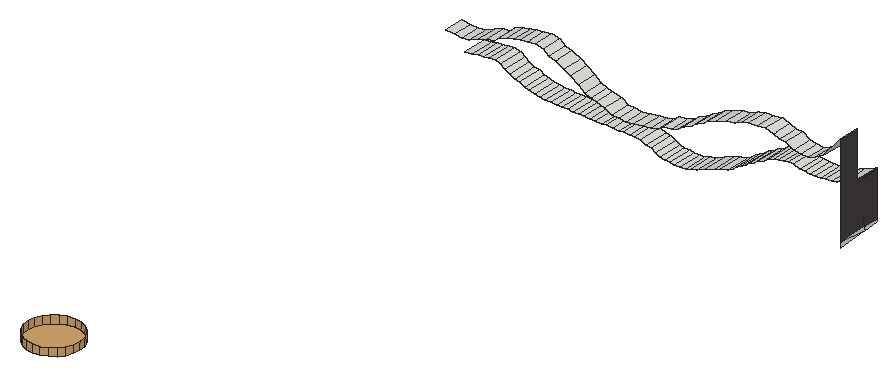
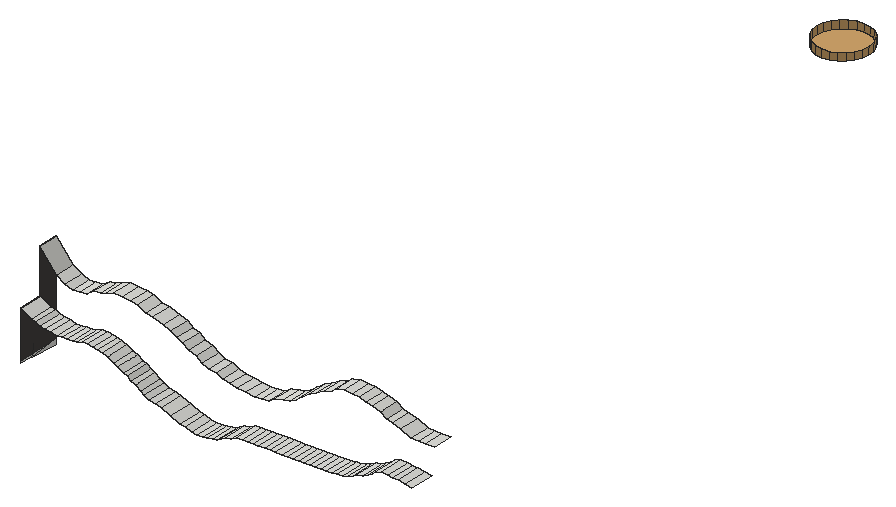
# SketchUp Ruby script. Lengths in inches.
U = 1.inch
M = Sketchup.active_model
def pt(a) = Geom::Point3d.new(a.map { |v| v * U })
def face(e, loops, mat)
  f = e.add_face(loops[0].map { |a| pt(a) })
  loops[1..].each { |l| e.add_face(l.map { |a| pt(a) }).erase! }
  f.material = f.back_material = mat if mat
  f
end
# faces: each face lists its corners as indices into pts; further lists are holes
def faces(e, pts, list, mat = nil) = list.each { |f| face(e, (f[0].is_a?(Array) ? f : [f]).map { |l| l.map { |i| pts[i] } }, mat) }
# xy, xz, yz: faces in a plane at the given z, y or x. An outline is a flat list of corners, or four numbers for a rectangle; further outlines are holes
def ring(l) = l.size == 4 ? [[l[0], l[1]], [l[2], l[1]], [l[2], l[3]], [l[0], l[3]]] : l.each_slice(2).to_a
def flat(e, list, mat, &to3) = list.each { |f| face(e, (f[0].is_a?(Array) ? f : [f]).map { |l| ring(l).map { |u, v| to3.(u, v) } }, mat) }
def xy(e, z, list, mat = nil) = flat(e, list, mat) { |x, y| [x, y, z] }
def xz(e, y, list, mat = nil) = flat(e, list, mat) { |x, z| [x, y, z] }
def yz(e, x, list, mat = nil) = flat(e, list, mat) { |y, z| [x, y, z] }
def lines(e, pts, list) = list.each { |a, b| e.add_line(pt(pts[a]), pt(pts[b])) }
# prism: a flat outline (further loops are holes) pulled along v
def prism(e, loops, v, mat = nil)
  f = face(e, loops, mat); d = Geom::Vector3d.new(v.map { |x| x * U })
  f.pushpull(f.normal.samedirection?(d) ? d.length : -d.length)
end
def box(e, o, s, mat = nil) = prism(e, [[o, [o[0] + s[0], o[1], o[2]], [o[0] + s[0], o[1] + s[1], o[2]], [o[0], o[1] + s[1], o[2]]]], [0, 0, s[2]], mat)
def at(x, y, z, deg = 0) = Geom::Transformation.translation(pt([x, y, z])) * Geom::Transformation.rotation(ORIGIN, Z_AXIS, deg.degrees)
def axes(o, x, y, z) = Geom::Transformation.new([*x, 0, *y, 0, *z, 0, *pt(o).to_a, 1])
def part(name) = M.definitions.add(name)
# library, detail: a bought-in or finely detailed component or shape, given as its bounding box
def library(name, o, s) = part(name).tap { |d| box(d.entities, o, s) }
def detail(e, o, s) = box(e.add_group.entities, o, s)
def put(e, d, t, mat = nil) = e.add_instance(d, t).tap { |i| i.material = mat if mat }
def group(e, t, mat = nil) = e.add_group.tap { |g| g.transformation = t; g.material = mat if mat }.entities
root = M.entities
M.materials.add("[Field Square Tile]").color = [211, 167, 108]
M.materials.add("[Granite Tile]1").color = [68, 65, 63]
xy(root,250.6875,[[2134.543,2328.207,2133.831,2328.3,2133.168,2328.575,2132.598,2329.012,2132.161,2329.582,2131.886,2330.245,2131.793,2330.957,2131.886,2331.668,2132.161,2332.332,2132.598,2332.901,2133.168,2333.338,2133.831,2333.613,2134.543,2333.707,2135.254,2333.613,2135.918,2333.338,2136.487,2332.901,2136.924,2332.332,2137.199,2331.668,2137.293,2330.957,2137.199,2330.245,2136.924,2329.582,2136.487,2329.012,2135.918,2328.575,2135.254,2328.3]],"[Field Square Tile]")
yz(root,2164.345,[[2396.678,240.932,2396.678,241.519,2399.776,241.17],[2399.81,241.167,2399.776,241.17,2399.809,241.173],[2399.776,241.17,2396.678,241.519,2399.769,241.519,2399.809,241.173],[2399.809,241.173,2399.769,241.519,2401.365,241.519,2401.365,241.293]])
yz(root,2164.345,[[2396.678,241.519,2396.678,251.165,2398.803,251.165,2398.803,246.426,2401.365,246.426,2401.365,241.519]],"[Granite Tile]1")
p = [[2144.767,2398.803,241.17],[2144.767,2401.365,241.17],[2145.237,2401.365,241.121],[2145.237,2398.803,241.121],[2145.843,2401.365,241.09],[2145.843,2398.803,241.09],
  [2146.41,2401.365,241.138],[2146.41,2398.803,241.138],[2147.05,2401.365,241.346],[2147.05,2398.803,241.346],[2143.769,2398.803,241.332],[2143.769,2401.365,241.332],
  [2144.237,2401.365,241.243],[2144.237,2398.803,241.243],[2143.35,2398.803,241.566],[2143.35,2401.365,241.566],[2147.641,2401.365,241.456],[2147.641,2398.803,241.456],
  [2148.576,2401.365,241.847],[2148.576,2398.803,241.847],[2142.844,2398.803,241.837],[2142.844,2401.365,241.837],[2142.271,2398.803,241.967],[2142.271,2401.365,241.967],
  [2149.581,2401.365,242.229],[2149.581,2398.803,242.229],[2141.69,2398.803,242.199],[2141.69,2401.365,242.199],[2141.064,2398.803,242.277],[2141.064,2401.365,242.277],
  [2150.142,2401.365,242.424],[2150.142,2398.803,242.424],[2135.217,2398.803,242.35],[2135.217,2401.365,242.35],[2135.799,2401.365,242.342],[2135.799,2398.803,242.342],
  [2136.381,2401.365,242.334],[2136.381,2398.803,242.334],[2136.963,2401.365,242.326],[2136.963,2398.803,242.326],[2137.683,2401.365,242.317],[2137.683,2398.803,242.317],
  [2138.153,2401.365,242.312],[2138.153,2398.803,242.312],[2138.794,2401.365,242.304],[2138.794,2398.803,242.304],[2139.458,2401.365,242.296],[2139.458,2398.803,242.296],
  [2139.91,2401.365,242.291],[2139.91,2398.803,242.291],[2140.548,2401.365,242.283],[2140.548,2398.803,242.283],[2131.735,2398.803,242.466],[2131.735,2401.365,242.466],
  [2132.311,2401.365,242.428],[2132.311,2398.803,242.428],[2132.89,2401.365,242.403],[2132.89,2398.803,242.403],[2133.47,2401.365,242.385],[2133.47,2398.803,242.385],
  [2134.052,2401.365,242.371],[2134.052,2398.803,242.371],[2134.634,2401.365,242.36],[2134.634,2398.803,242.36],[2150.86,2401.365,242.605],[2150.86,2398.803,242.605],
  [2130.607,2398.803,242.599],[2130.607,2401.365,242.599],[2131.167,2401.365,242.518],[2131.167,2398.803,242.518],[2130.054,2398.803,242.75],[2130.054,2401.365,242.75],
  [2151.373,2401.365,242.907],[2151.373,2398.803,242.907],[2129.566,2398.803,242.921],[2129.566,2401.365,242.921],[2129.075,2398.803,243.216],[2129.075,2401.365,243.216],
  [2151.745,2401.365,243.144],[2151.745,2398.803,243.144],[2152.294,2401.365,243.516],[2152.294,2398.803,243.516],[2128.527,2398.803,243.332],[2128.527,2401.365,243.332],
  [2127.982,2398.803,243.589],[2127.982,2401.365,243.589],[2152.768,2401.365,243.711],[2152.768,2398.803,243.711],[2127.501,2398.803,243.88],[2127.501,2401.365,243.88],
  [2153.099,2401.365,244.02],[2153.099,2398.803,244.02],[2127.124,2398.803,244.194],[2127.124,2401.365,244.194],[2123.336,2398.803,243.992],[2123.336,2401.365,243.992],
  [2124.039,2401.365,244.076],[2124.039,2398.803,244.076],[2153.543,2401.365,244.206],[2153.543,2398.803,244.206],[2124.738,2401.365,244.207],[2124.738,2398.803,244.207],
  [2125.323,2401.365,244.266],[2125.323,2398.803,244.266],[2126.527,2398.803,244.387],[2126.527,2401.365,244.387],[2154.132,2401.365,244.569],[2154.132,2398.803,244.569],
  [2125.864,2401.365,244.296],[2125.864,2398.803,244.296],[2154.602,2401.365,244.757],[2154.602,2398.803,244.757],[2155.219,2401.365,245.125],[2155.219,2398.803,245.125],
  [2140.415,2396.678,245.064],[2140.415,2398.803,245.064],[2141.125,2398.803,244.949],[2141.125,2396.678,244.949],[2141.839,2398.803,244.867],[2141.839,2396.678,244.867],
  [2142.745,2398.803,245.007],[2142.745,2396.678,245.007],[2143.689,2398.803,245.121],[2143.689,2396.678,245.121],[2139.702,2396.678,245.459],[2139.702,2398.803,245.459],
  [2144.454,2398.803,245.254],[2144.454,2396.678,245.254],[2155.723,2401.365,245.32],[2155.723,2398.803,245.32],[2159.424,2398.803,245.272],[2159.424,2401.365,245.272],
  [2159.982,2401.365,245.235],[2159.982,2398.803,245.235],[2160.536,2401.365,245.216],[2160.536,2398.803,245.216],[2161.101,2401.365,245.34],[2161.101,2398.803,245.34],
  [2145.206,2398.803,245.41],[2145.206,2396.678,245.41],[2156.205,2401.365,245.411],[2156.205,2398.803,245.411],[2157.771,2398.803,245.552],[2157.771,2401.365,245.552],
  [2158.379,2401.365,245.346],[2158.379,2398.803,245.346],[2158.873,2401.365,245.309],[2158.873,2398.803,245.309],[2161.733,2401.365,245.423],[2161.733,2398.803,245.423],
  [2145.84,2398.803,245.775],[2145.84,2396.678,245.775],[2156.753,2401.365,245.481],[2156.753,2398.803,245.481],[2162.311,2401.365,245.516],[2162.311,2398.803,245.516],
  [2138.827,2396.678,245.671],[2138.827,2398.803,245.671],[2157.235,2401.365,245.59],[2157.235,2398.803,245.59],[2162.691,2401.365,245.763],[2162.691,2398.803,245.763],
  [2138.152,2396.678,245.834],[2138.152,2398.803,245.834],[2137.564,2396.678,246.129],[2137.564,2398.803,246.129],[2146.636,2398.803,245.88],[2146.636,2396.678,245.88],
  [2163.16,2401.365,245.896],[2163.16,2398.803,245.896],[2147.349,2398.803,246.16],[2147.349,2396.678,246.16],[2164.345,2401.365,246.426],[2164.345,2398.803,246.426],
  [2136.933,2396.678,246.633],[2136.933,2398.803,246.633],[2147.946,2398.803,246.573],[2147.946,2396.678,246.573],[2136.119,2396.678,247.185],[2136.119,2398.803,247.185],
  [2148.736,2398.803,246.902],[2148.736,2396.678,246.902],[2123.942,2396.678,246.79],[2123.942,2398.803,246.79],[2124.721,2398.803,246.747],[2124.721,2396.678,246.747],
  [2125.468,2398.803,246.831],[2125.468,2396.678,246.831],[2122.988,2396.678,246.838],[2122.988,2398.803,246.838],[2126.51,2398.803,247.251],[2126.51,2396.678,247.251],
  [2149.338,2398.803,247.347],[2149.338,2396.678,247.347],[2135.407,2396.678,247.553],[2135.407,2398.803,247.553],[2127.384,2398.803,247.546],[2127.384,2396.678,247.546],
  [2150.012,2398.803,247.615],[2150.012,2396.678,247.615],[2128.046,2398.803,247.657],[2128.046,2396.678,247.657],[2134.516,2396.678,248.059],[2134.516,2398.803,248.059],
  [2150.599,2398.803,248.057],[2150.599,2396.678,248.057],[2128.679,2398.803,248.162],[2128.679,2396.678,248.162],[2133.825,2396.678,248.257],[2133.825,2398.803,248.257],
  [2151.364,2398.803,248.322],[2151.364,2396.678,248.322],[2129.473,2398.803,248.408],[2129.473,2396.678,248.408],[2160.161,2396.678,248.295],[2160.161,2398.803,248.295],
  [2160.87,2398.803,248.218],[2160.87,2396.678,248.218],[2161.687,2398.803,248.558],[2161.687,2396.678,248.558],[2133.294,2396.678,248.687],[2133.294,2398.803,248.687],
  [2152.475,2398.803,248.655],[2152.475,2396.678,248.655],[2159.45,2396.678,248.42],[2159.45,2398.803,248.42],[2130.172,2398.803,248.521],[2130.172,2396.678,248.521],
  [2158.653,2396.678,248.895],[2158.653,2398.803,248.895],[2130.866,2398.803,248.723],[2130.866,2396.678,248.723],[2162.622,2398.803,249.022],[2162.622,2396.678,249.022],
  [2131.565,2398.803,248.801],[2131.565,2396.678,248.801],[2132.462,2396.678,248.851],[2132.462,2398.803,248.851],[2153.248,2398.803,248.795],[2153.248,2396.678,248.795],
  [2154.111,2398.803,249.194],[2154.111,2396.678,249.194],[2157.949,2396.678,248.962],[2157.949,2398.803,248.962],[2157.31,2396.678,249.206],[2157.31,2398.803,249.206],
  [2164.345,2398.803,251.165],[2164.345,2396.678,251.165],[2154.784,2398.803,249.323],[2154.784,2396.678,249.323],[2156.565,2396.678,249.478],[2156.565,2398.803,249.478],
  [2155.707,2398.803,249.406],[2155.707,2396.678,249.406],[2134.543,2328.207,251.5],[2133.831,2328.3,251.5],[2133.831,2328.3,250.6875],[2134.543,2328.207,250.6875],
  [2135.254,2328.3,251.5],[2135.254,2328.3,250.6875],[2133.168,2328.575,251.5],[2133.168,2328.575,250.6875],[2135.918,2328.575,251.5],[2135.918,2328.575,250.6875],
  [2132.598,2329.012,251.5],[2132.598,2329.012,250.6875],[2136.487,2329.012,251.5],[2136.487,2329.012,250.6875],[2132.161,2329.582,251.5],[2132.161,2329.582,250.6875],
  [2136.924,2329.582,251.5],[2136.924,2329.582,250.6875],[2131.886,2330.245,251.5],[2131.886,2330.245,250.6875],[2137.199,2330.245,251.5],[2137.199,2330.245,250.6875],
  [2131.793,2330.957,251.5],[2131.793,2330.957,250.6875],[2137.293,2330.957,251.5],[2137.293,2330.957,250.6875],[2131.886,2331.668,251.5],[2131.886,2331.668,250.6875],
  [2137.199,2331.668,251.5],[2137.199,2331.668,250.6875],[2132.161,2332.332,251.5],[2132.161,2332.332,250.6875],[2136.924,2332.332,251.5],[2136.924,2332.332,250.6875],
  [2132.598,2332.901,251.5],[2132.598,2332.901,250.6875],[2136.487,2332.901,251.5],[2136.487,2332.901,250.6875],[2133.168,2333.338,251.5],[2133.168,2333.338,250.6875],
  [2135.918,2333.338,251.5],[2135.918,2333.338,250.6875],[2133.831,2333.613,251.5],[2133.831,2333.613,250.6875],[2135.254,2333.613,251.5],[2135.254,2333.613,250.6875],
  [2134.543,2333.707,251.5],[2134.543,2333.707,250.6875],[2164.345,2400.588,246.171],[2164.345,2399.573,246.265],[2164.345,2401.365,246.273],[2164.345,2399.769,241.519],
  [2164.345,2399.667,242.384]]
faces(root,p,[[0,1,2,3],[3,2,4,5],[5,4,6,7],[7,6,8,9],[10,11,12,13],[13,12,1,0],[14,15,11,10],[9,8,16,17],
  [17,16,18,19],[20,21,15,14],[22,23,21,20],[19,18,24,25],[26,27,23,22],[28,29,27,26],[25,24,30,31],[32,33,34,35],
  [35,34,36,37],[37,36,38,39],[39,38,40,41],[41,40,42,43],[43,42,44,45],[45,44,46,47],[47,46,48,49],[49,48,50,51],
  [51,50,29,28],[52,53,54,55],[55,54,56,57],[57,56,58,59],[59,58,60,61],[61,60,62,63],[63,62,33,32],[31,30,64,65],
  [66,67,68,69],[69,68,53,52],[70,71,67,66],[65,64,72,73],[74,75,71,70],[76,77,75,74],[73,72,78,79],[79,78,80,81],
  [82,83,77,76],[84,85,83,82],[81,80,86,87],[88,89,85,84],[87,86,90,91],[92,93,89,88],[94,95,96,97],[91,90,98,99],
  [97,96,100,101],[101,100,102,103],[104,105,93,92],[99,98,106,107],[103,102,108,109],[109,108,105,104],[107,106,110,111],[111,110,112,113],
  [114,115,116,117],[117,116,118,119],[119,118,120,121],[121,120,122,123],[124,125,115,114],[123,122,126,127],[113,112,128,129],[130,131,132,133],
  [133,132,134,135],[135,134,136,137],[127,126,138,139],[129,128,140,141],[142,143,144,145],[145,144,146,147],[147,146,131,130],[137,136,148,149],
  [139,138,150,151],[141,140,152,153],[149,148,154,155],[156,157,125,124],[153,152,158,159],[155,154,160,161],[159,158,143,142],[162,163,157,156],
  [164,165,163,162],[151,150,166,167],[161,160,168,169],[167,166,170,171],[169,168,172,173],[174,175,165,164],[171,170,176,177],[178,179,175,174],
  [177,176,180,181],[182,183,184,185],[185,184,186,187],[188,189,183,182],[187,186,190,191],[181,180,192,193],[194,195,179,178],[191,190,196,197],
  [193,192,198,199],[197,196,200,201],[202,203,195,194],[199,198,204,205],[201,200,206,207],[208,209,203,202],[205,204,210,211],[207,206,212,213],
  [214,215,216,217],[217,216,218,219],[220,221,209,208],[211,210,222,223],[224,225,215,214],[213,212,226,227],[228,229,225,224],[227,226,230,231],
  [219,218,232,233],[231,230,234,235],[236,237,221,220],[223,222,238,239],[235,234,237,236],[239,238,240,241],[242,243,229,228],[244,245,243,242],
  [233,232,246,247],[241,240,248,249],[250,251,245,244],[249,248,252,253],[253,252,251,250]])
faces(root,p,[[254,255,256,257],[258,254,257,259],[255,260,261,256],[262,258,259,263],[260,264,265,261],[266,262,263,267],[264,268,269,265],[270,266,267,271],
  [268,272,273,269],[274,270,271,275],[272,276,277,273],[278,274,275,279],[276,280,281,277],[282,278,279,283],[280,284,285,281],[286,282,283,287],
  [284,288,289,285],[290,286,287,291],[288,292,293,289],[294,290,291,295],[292,296,297,293],[298,294,295,299],[296,300,301,297],[300,298,299,301]],"[Field Square Tile]")
lines(root,p,[[302,303],[304,302],[305,306]])
